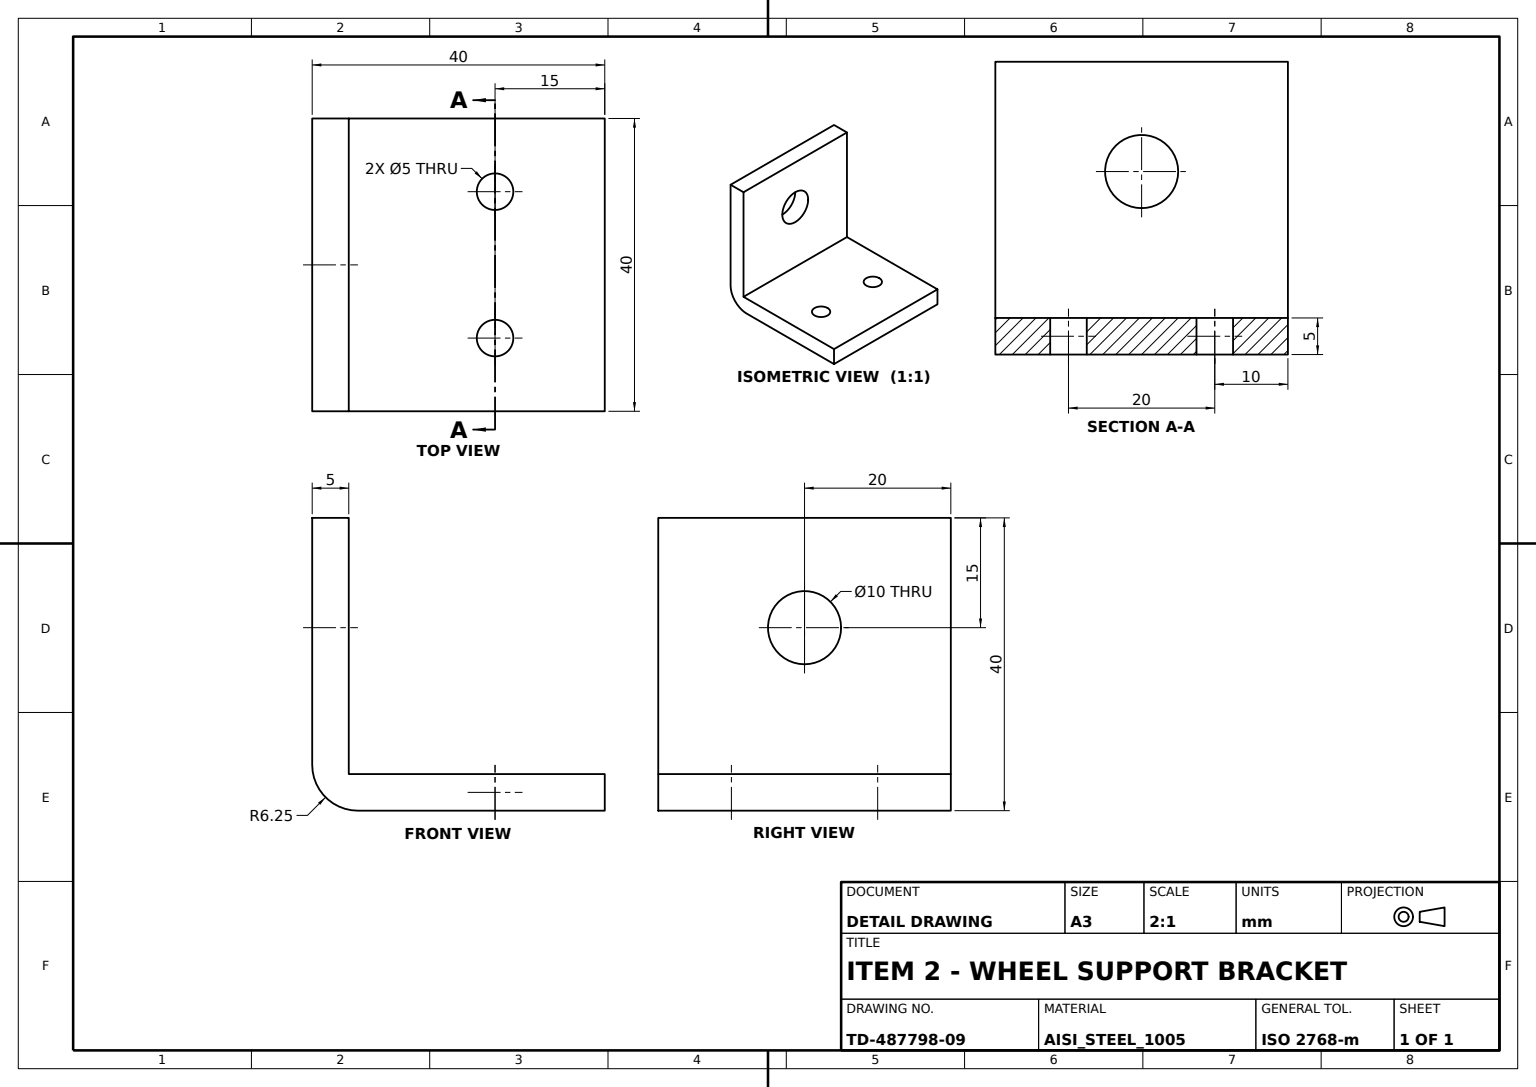
ISO-10303-21;
HEADER;
FILE_DESCRIPTION((''),'2;1');
FILE_NAME('','',(''),(''),'','','');
FILE_SCHEMA(('AUTOMOTIVE_DESIGN'));
ENDSEC;
DATA;
#1=APPLICATION_CONTEXT('');
#2=PRODUCT_CONTEXT('',#1,'mechanical');
#3=PRODUCT('','','',(#2));
#4=PRODUCT_DEFINITION_FORMATION('','',#3);
#5=PRODUCT_DEFINITION_CONTEXT('',#1,'design');
#6=PRODUCT_DEFINITION('','',#4,#5);
#7=PRODUCT_DEFINITION_SHAPE('','',#6);
#8=(LENGTH_UNIT()NAMED_UNIT(*)SI_UNIT(.MILLI.,.METRE.));
#9=(NAMED_UNIT(*)PLANE_ANGLE_UNIT()SI_UNIT($,.RADIAN.));
#10=(NAMED_UNIT(*)SI_UNIT($,.STERADIAN.)SOLID_ANGLE_UNIT());
#11=UNCERTAINTY_MEASURE_WITH_UNIT(LENGTH_MEASURE(0.005),#8,'distance_accuracy_value','');
#12=(GEOMETRIC_REPRESENTATION_CONTEXT(3)GLOBAL_UNCERTAINTY_ASSIGNED_CONTEXT((#11))GLOBAL_UNIT_ASSIGNED_CONTEXT((#8,#9,#10))REPRESENTATION_CONTEXT('',''));
#13=CARTESIAN_POINT('',(27.5,-10.,0.));
#14=VERTEX_POINT('',#13);
#15=CARTESIAN_POINT('',(25.,-10.,0.));
#16=DIRECTION('',(0.,0.,1.));
#17=DIRECTION('',(1.,0.,0.));
#18=AXIS2_PLACEMENT_3D('',#15,#16,#17);
#19=CIRCLE('',#18,2.5);
#20=EDGE_CURVE('',#14,#14,#19,.F.);
#21=ORIENTED_EDGE('',*,*,#20,.T.);
#22=EDGE_LOOP('',(#21));
#23=FACE_BOUND('',#22,.T.);
#24=CARTESIAN_POINT('',(25.,-7.5,5.));
#25=VERTEX_POINT('',#24);
#26=CARTESIAN_POINT('',(25.,-10.,5.));
#27=DIRECTION('',(0.,0.,-1.));
#28=DIRECTION('',(0.,1.,0.));
#29=AXIS2_PLACEMENT_3D('',#26,#27,#28);
#30=CIRCLE('',#29,2.5);
#31=EDGE_CURVE('',#25,#25,#30,.T.);
#32=ORIENTED_EDGE('',*,*,#31,.F.);
#33=EDGE_LOOP('',(#32));
#34=FACE_BOUND('',#33,.T.);
#35=CARTESIAN_POINT('',(25.,-10.,-5.));
#36=AXIS2_PLACEMENT_3D('',#35,#16,#17);
#37=CYLINDRICAL_SURFACE('',#36,2.5);
#38=ADVANCED_FACE('',(#23,#34),#37,.F.);
#39=CARTESIAN_POINT('',(5.,20.,40.));
#40=VERTEX_POINT('',#39);
#41=CARTESIAN_POINT('',(0.,20.,40.));
#42=VERTEX_POINT('',#41);
#43=DIRECTION('',(-1.,0.,0.));
#44=VECTOR('',#43,1000.);
#45=LINE('',#39,#44);
#46=EDGE_CURVE('',#40,#42,#45,.T.);
#47=ORIENTED_EDGE('',*,*,#46,.T.);
#48=CARTESIAN_POINT('',(0.,-20.,40.));
#49=VERTEX_POINT('',#48);
#50=VECTOR('',#28,1000.);
#51=LINE('',#48,#50);
#52=EDGE_CURVE('',#49,#42,#51,.T.);
#53=ORIENTED_EDGE('',*,*,#52,.F.);
#54=CARTESIAN_POINT('',(5.,-20.,40.));
#55=VERTEX_POINT('',#54);
#56=LINE('',#54,#44);
#57=EDGE_CURVE('',#55,#49,#56,.T.);
#58=ORIENTED_EDGE('',*,*,#57,.F.);
#59=LINE('',#54,#50);
#60=EDGE_CURVE('',#55,#40,#59,.T.);
#61=ORIENTED_EDGE('',*,*,#60,.T.);
#62=EDGE_LOOP('',(#47,#53,#58,#61));
#63=FACE_BOUND('',#62,.T.);
#64=AXIS2_PLACEMENT_3D('',#54,#27,#43);
#65=PLANE('',#64);
#66=ADVANCED_FACE('',(#63),#65,.F.);
#67=CARTESIAN_POINT('',(5.,5.,25.));
#68=VERTEX_POINT('',#67);
#69=CARTESIAN_POINT('',(5.,0.,25.));
#70=AXIS2_PLACEMENT_3D('',#69,#17,#28);
#71=CIRCLE('',#70,5.);
#72=EDGE_CURVE('',#68,#68,#71,.T.);
#73=ORIENTED_EDGE('',*,*,#72,.F.);
#74=EDGE_LOOP('',(#73));
#75=FACE_BOUND('',#74,.T.);
#76=CARTESIAN_POINT('',(5.,-20.,5.));
#77=VERTEX_POINT('',#76);
#78=VECTOR('',#16,1000.);
#79=LINE('',#76,#78);
#80=EDGE_CURVE('',#77,#55,#79,.T.);
#81=ORIENTED_EDGE('',*,*,#80,.F.);
#82=CARTESIAN_POINT('',(5.,20.,5.));
#83=VERTEX_POINT('',#82);
#84=LINE('',#76,#50);
#85=EDGE_CURVE('',#77,#83,#84,.T.);
#86=ORIENTED_EDGE('',*,*,#85,.T.);
#87=LINE('',#82,#78);
#88=EDGE_CURVE('',#83,#40,#87,.T.);
#89=ORIENTED_EDGE('',*,*,#88,.T.);
#90=ORIENTED_EDGE('',*,*,#60,.F.);
#91=EDGE_LOOP('',(#81,#86,#89,#90));
#92=FACE_BOUND('',#91,.T.);
#93=AXIS2_PLACEMENT_3D('',#76,#43,#16);
#94=PLANE('',#93);
#95=ADVANCED_FACE('',(#75,#92),#94,.F.);
#96=CARTESIAN_POINT('',(40.,-20.,5.));
#97=VERTEX_POINT('',#96);
#98=CARTESIAN_POINT('',(40.,20.,5.));
#99=VERTEX_POINT('',#98);
#100=LINE('',#96,#50);
#101=EDGE_CURVE('',#97,#99,#100,.T.);
#102=ORIENTED_EDGE('',*,*,#101,.F.);
#103=CARTESIAN_POINT('',(40.,-20.,0.));
#104=VERTEX_POINT('',#103);
#105=LINE('',#103,#78);
#106=EDGE_CURVE('',#104,#97,#105,.T.);
#107=ORIENTED_EDGE('',*,*,#106,.F.);
#108=CARTESIAN_POINT('',(40.,20.,0.));
#109=VERTEX_POINT('',#108);
#110=LINE('',#103,#50);
#111=EDGE_CURVE('',#104,#109,#110,.T.);
#112=ORIENTED_EDGE('',*,*,#111,.T.);
#113=LINE('',#108,#78);
#114=EDGE_CURVE('',#109,#99,#113,.T.);
#115=ORIENTED_EDGE('',*,*,#114,.T.);
#116=EDGE_LOOP('',(#102,#107,#112,#115));
#117=FACE_BOUND('',#116,.T.);
#118=AXIS2_PLACEMENT_3D('',#103,#43,#16);
#119=PLANE('',#118);
#120=ADVANCED_FACE('',(#117),#119,.F.);
#121=CARTESIAN_POINT('',(0.,0.,20.));
#122=VERTEX_POINT('',#121);
#123=CARTESIAN_POINT('',(0.,0.,25.));
#124=AXIS2_PLACEMENT_3D('',#123,#17,#27);
#125=CIRCLE('',#124,5.);
#126=EDGE_CURVE('',#122,#122,#125,.T.);
#127=ORIENTED_EDGE('',*,*,#126,.F.);
#128=EDGE_LOOP('',(#127));
#129=FACE_BOUND('',#128,.T.);
#130=ORIENTED_EDGE('',*,*,#72,.T.);
#131=EDGE_LOOP('',(#130));
#132=FACE_BOUND('',#131,.T.);
#133=CARTESIAN_POINT('',(-15.,0.,25.));
#134=AXIS2_PLACEMENT_3D('',#133,#17,#27);
#135=CYLINDRICAL_SURFACE('',#134,5.);
#136=ADVANCED_FACE('',(#129,#132),#135,.F.);
#137=ORIENTED_EDGE('',*,*,#101,.T.);
#138=LINE('',#98,#44);
#139=EDGE_CURVE('',#99,#83,#138,.T.);
#140=ORIENTED_EDGE('',*,*,#139,.T.);
#141=ORIENTED_EDGE('',*,*,#85,.F.);
#142=LINE('',#96,#44);
#143=EDGE_CURVE('',#97,#77,#142,.T.);
#144=ORIENTED_EDGE('',*,*,#143,.F.);
#145=EDGE_LOOP('',(#137,#140,#141,#144));
#146=FACE_BOUND('',#145,.T.);
#147=ORIENTED_EDGE('',*,*,#31,.T.);
#148=EDGE_LOOP('',(#147));
#149=FACE_BOUND('',#148,.T.);
#150=CARTESIAN_POINT('',(25.,12.5,5.));
#151=VERTEX_POINT('',#150);
#152=CARTESIAN_POINT('',(25.,10.,5.));
#153=AXIS2_PLACEMENT_3D('',#152,#27,#28);
#154=CIRCLE('',#153,2.5);
#155=EDGE_CURVE('',#151,#151,#154,.T.);
#156=ORIENTED_EDGE('',*,*,#155,.T.);
#157=EDGE_LOOP('',(#156));
#158=FACE_BOUND('',#157,.T.);
#159=AXIS2_PLACEMENT_3D('',#96,#27,#43);
#160=PLANE('',#159);
#161=ADVANCED_FACE('',(#146,#149,#158),#160,.F.);
#162=CARTESIAN_POINT('',(6.25,-20.,0.));
#163=VERTEX_POINT('',#162);
#164=CARTESIAN_POINT('',(6.25,20.,0.));
#165=VERTEX_POINT('',#164);
#166=LINE('',#162,#50);
#167=EDGE_CURVE('',#163,#165,#166,.T.);
#168=ORIENTED_EDGE('',*,*,#167,.F.);
#169=CARTESIAN_POINT('',(0.,-20.,6.25));
#170=VERTEX_POINT('',#169);
#171=CARTESIAN_POINT('',(6.25,-20.,6.25));
#172=DIRECTION('',(0.,-1.,0.));
#173=AXIS2_PLACEMENT_3D('',#171,#172,#27);
#174=CIRCLE('',#173,6.25);
#175=EDGE_CURVE('',#170,#163,#174,.T.);
#176=ORIENTED_EDGE('',*,*,#175,.F.);
#177=CARTESIAN_POINT('',(0.,20.,6.25));
#178=VERTEX_POINT('',#177);
#179=LINE('',#169,#50);
#180=EDGE_CURVE('',#178,#170,#179,.F.);
#181=ORIENTED_EDGE('',*,*,#180,.F.);
#182=CARTESIAN_POINT('',(6.25,20.,6.25));
#183=AXIS2_PLACEMENT_3D('',#182,#172,#27);
#184=CIRCLE('',#183,6.25);
#185=EDGE_CURVE('',#165,#178,#184,.F.);
#186=ORIENTED_EDGE('',*,*,#185,.F.);
#187=EDGE_LOOP('',(#168,#176,#181,#186));
#188=FACE_BOUND('',#187,.T.);
#189=AXIS2_PLACEMENT_3D('',#171,#28,#16);
#190=CYLINDRICAL_SURFACE('',#189,6.25);
#191=ADVANCED_FACE('',(#188),#190,.T.);
#192=CARTESIAN_POINT('',(27.5,10.,0.));
#193=VERTEX_POINT('',#192);
#194=CARTESIAN_POINT('',(25.,10.,0.));
#195=AXIS2_PLACEMENT_3D('',#194,#16,#17);
#196=CIRCLE('',#195,2.5);
#197=EDGE_CURVE('',#193,#193,#196,.F.);
#198=ORIENTED_EDGE('',*,*,#197,.T.);
#199=EDGE_LOOP('',(#198));
#200=FACE_BOUND('',#199,.T.);
#201=ORIENTED_EDGE('',*,*,#155,.F.);
#202=EDGE_LOOP('',(#201));
#203=FACE_BOUND('',#202,.T.);
#204=CARTESIAN_POINT('',(25.,10.,-5.));
#205=AXIS2_PLACEMENT_3D('',#204,#16,#17);
#206=CYLINDRICAL_SURFACE('',#205,2.5);
#207=ADVANCED_FACE('',(#200,#203),#206,.F.);
#208=ORIENTED_EDGE('',*,*,#143,.T.);
#209=ORIENTED_EDGE('',*,*,#80,.T.);
#210=ORIENTED_EDGE('',*,*,#57,.T.);
#211=VECTOR('',#27,1000.);
#212=LINE('',#48,#211);
#213=EDGE_CURVE('',#49,#170,#212,.T.);
#214=ORIENTED_EDGE('',*,*,#213,.T.);
#215=ORIENTED_EDGE('',*,*,#175,.T.);
#216=CARTESIAN_POINT('',(0.,-20.,0.));
#217=VECTOR('',#17,1000.);
#218=LINE('',#216,#217);
#219=EDGE_CURVE('',#163,#104,#218,.T.);
#220=ORIENTED_EDGE('',*,*,#219,.T.);
#221=ORIENTED_EDGE('',*,*,#106,.T.);
#222=EDGE_LOOP('',(#208,#209,#210,#214,#215,#220,#221));
#223=FACE_BOUND('',#222,.T.);
#224=AXIS2_PLACEMENT_3D('',#216,#172,#27);
#225=PLANE('',#224);
#226=ADVANCED_FACE('',(#223),#225,.T.);
#227=ORIENTED_EDGE('',*,*,#46,.F.);
#228=ORIENTED_EDGE('',*,*,#88,.F.);
#229=ORIENTED_EDGE('',*,*,#139,.F.);
#230=ORIENTED_EDGE('',*,*,#114,.F.);
#231=CARTESIAN_POINT('',(0.,20.,0.));
#232=LINE('',#231,#217);
#233=EDGE_CURVE('',#165,#109,#232,.T.);
#234=ORIENTED_EDGE('',*,*,#233,.F.);
#235=ORIENTED_EDGE('',*,*,#185,.T.);
#236=LINE('',#41,#211);
#237=EDGE_CURVE('',#42,#178,#236,.T.);
#238=ORIENTED_EDGE('',*,*,#237,.F.);
#239=EDGE_LOOP('',(#227,#228,#229,#230,#234,#235,#238));
#240=FACE_BOUND('',#239,.T.);
#241=AXIS2_PLACEMENT_3D('',#231,#172,#27);
#242=PLANE('',#241);
#243=ADVANCED_FACE('',(#240),#242,.F.);
#244=ORIENTED_EDGE('',*,*,#197,.F.);
#245=EDGE_LOOP('',(#244));
#246=FACE_BOUND('',#245,.T.);
#247=ORIENTED_EDGE('',*,*,#233,.T.);
#248=ORIENTED_EDGE('',*,*,#111,.F.);
#249=ORIENTED_EDGE('',*,*,#219,.F.);
#250=ORIENTED_EDGE('',*,*,#167,.T.);
#251=EDGE_LOOP('',(#247,#248,#249,#250));
#252=FACE_BOUND('',#251,.T.);
#253=ORIENTED_EDGE('',*,*,#20,.F.);
#254=EDGE_LOOP('',(#253));
#255=FACE_BOUND('',#254,.T.);
#256=AXIS2_PLACEMENT_3D('',#216,#16,#17);
#257=PLANE('',#256);
#258=ADVANCED_FACE('',(#246,#252,#255),#257,.F.);
#259=ORIENTED_EDGE('',*,*,#126,.T.);
#260=EDGE_LOOP('',(#259));
#261=FACE_BOUND('',#260,.T.);
#262=ORIENTED_EDGE('',*,*,#237,.T.);
#263=ORIENTED_EDGE('',*,*,#180,.T.);
#264=ORIENTED_EDGE('',*,*,#213,.F.);
#265=ORIENTED_EDGE('',*,*,#52,.T.);
#266=EDGE_LOOP('',(#262,#263,#264,#265));
#267=FACE_BOUND('',#266,.T.);
#268=AXIS2_PLACEMENT_3D('',#48,#17,#27);
#269=PLANE('',#268);
#270=ADVANCED_FACE('',(#261,#267),#269,.F.);
#271=CLOSED_SHELL('',(#38,#66,#95,#120,#136,#161,#191,#207,#226,#243,#258,#270));
#272=MANIFOLD_SOLID_BREP('',#271);
#273=ADVANCED_BREP_SHAPE_REPRESENTATION('',(#272),#12);
#274=SHAPE_DEFINITION_REPRESENTATION(#7,#273);
ENDSEC;
END-ISO-10303-21;
